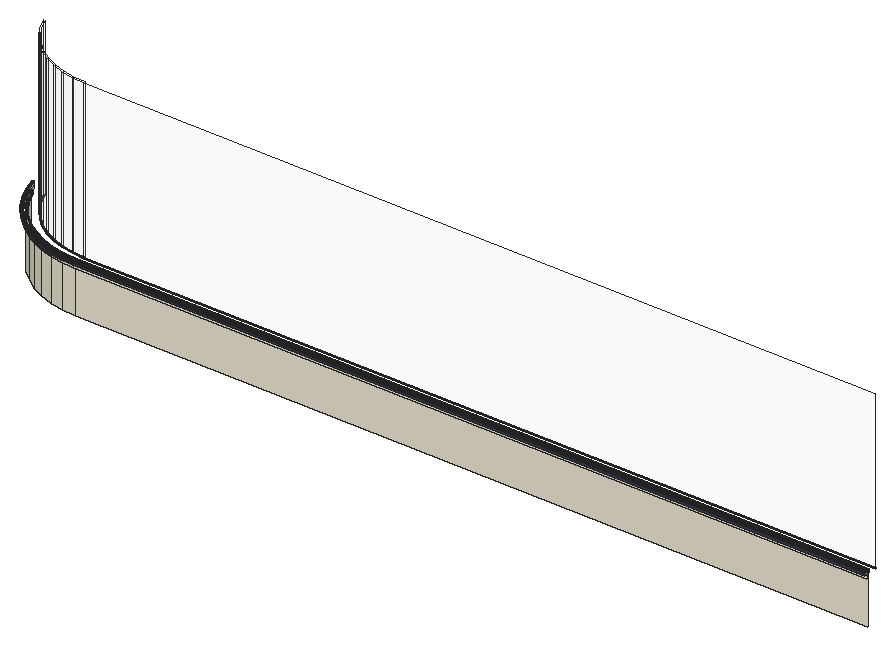
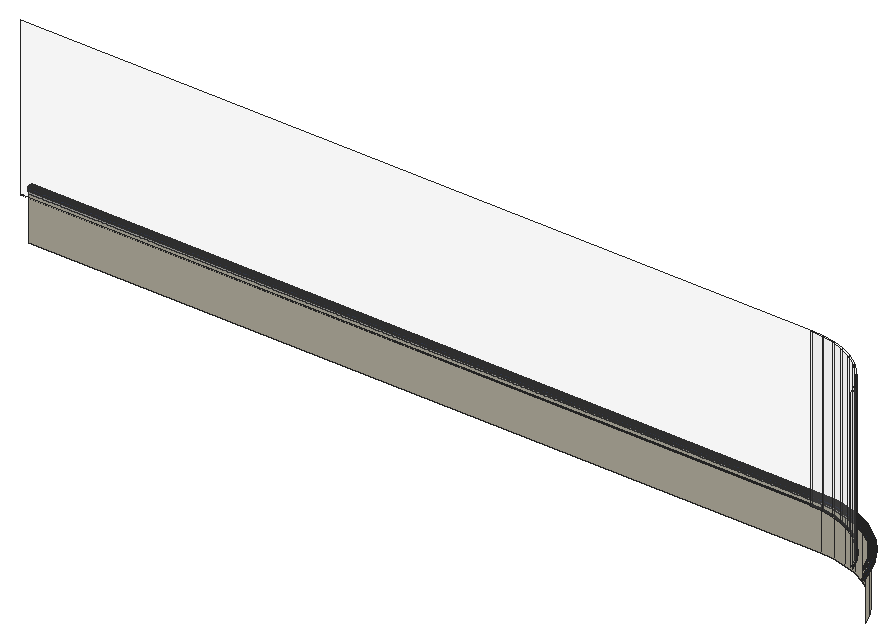
# SketchUp Ruby script. Lengths in inches.
U = 1.inch
M = Sketchup.active_model
def pt(a) = Geom::Point3d.new(a.map { |v| v * U })
def face(e, loops, mat)
  f = e.add_face(loops[0].map { |a| pt(a) })
  loops[1..].each { |l| e.add_face(l.map { |a| pt(a) }).erase! }
  f.material = f.back_material = mat if mat
  f
end
# faces: each face lists its corners as indices into pts; further lists are holes
def faces(e, pts, list, mat = nil) = list.each { |f| face(e, (f[0].is_a?(Array) ? f : [f]).map { |l| l.map { |i| pts[i] } }, mat) }
# xy, xz, yz: faces in a plane at the given z, y or x. An outline is a flat list of corners, or four numbers for a rectangle; further outlines are holes
def ring(l) = l.size == 4 ? [[l[0], l[1]], [l[2], l[1]], [l[2], l[3]], [l[0], l[3]]] : l.each_slice(2).to_a
def flat(e, list, mat, &to3) = list.each { |f| face(e, (f[0].is_a?(Array) ? f : [f]).map { |l| ring(l).map { |u, v| to3.(u, v) } }, mat) }
def xy(e, z, list, mat = nil) = flat(e, list, mat) { |x, y| [x, y, z] }
def xz(e, y, list, mat = nil) = flat(e, list, mat) { |x, z| [x, y, z] }
def yz(e, x, list, mat = nil) = flat(e, list, mat) { |y, z| [x, y, z] }
def lines(e, pts, list) = list.each { |a, b| e.add_line(pt(pts[a]), pt(pts[b])) }
# prism: a flat outline (further loops are holes) pulled along v
def prism(e, loops, v, mat = nil)
  f = face(e, loops, mat); d = Geom::Vector3d.new(v.map { |x| x * U })
  f.pushpull(f.normal.samedirection?(d) ? d.length : -d.length)
end
def box(e, o, s, mat = nil) = prism(e, [[o, [o[0] + s[0], o[1], o[2]], [o[0] + s[0], o[1] + s[1], o[2]], [o[0], o[1] + s[1], o[2]]]], [0, 0, s[2]], mat)
def at(x, y, z, deg = 0) = Geom::Transformation.translation(pt([x, y, z])) * Geom::Transformation.rotation(ORIGIN, Z_AXIS, deg.degrees)
def axes(o, x, y, z) = Geom::Transformation.new([*x, 0, *y, 0, *z, 0, *pt(o).to_a, 1])
def part(name) = M.definitions.add(name)
# library, detail: a bought-in or finely detailed component or shape, given as its bounding box
def library(name, o, s) = part(name).tap { |d| box(d.entities, o, s) }
def detail(e, o, s) = box(e.add_group.entities, o, s)
def put(e, d, t, mat = nil) = e.add_instance(d, t).tap { |i| i.material = mat if mat }
def group(e, t, mat = nil) = e.add_group.tap { |g| g.transformation = t; g.material = mat if mat }.entities
root = M.entities
M.materials.add("0360 AP 9644 Monsoon Midnight-N").color = [56, 67, 95]
M.materials.add("0905 AP 7844 MILD YELLOW").color = [242, 237, 215]
M.materials.add("Glass Clear 001").color = [246, 246, 246]
M.materials["Glass Clear 001"].alpha = 0.1
xz(root,29.01,[[57,132.5625,238.5625,132.625],[57,132.625,238.5625,132.8125]],"0360 AP 9644 Monsoon Midnight-N")
xz(root,29.09,[[57,132.5625,238.5625,132.625]])
xz(root,29.09,[[57,132,238.5625,132.5625],[57,132.625,238.5625,132.8125]],"0360 AP 9644 Monsoon Midnight-N")
xz(root,29.45,[[57,132,238.5625,132.625]])
xz(root,29.45,[[57,132.625,238.5625,132.8125]],"0360 AP 9644 Monsoon Midnight-N")
xz(root,29.45,[[57,131.3125,238.5625,132]],"0905 AP 7844 MILD YELLOW")
xz(root,29.53,[[57,132.625,238.5625,132.8125]],"0360 AP 9644 Monsoon Midnight-N")
xz(root,29.9375,[[57,131.3125,238.5625,132.625]])
xz(root,29.9375,[[57,132.625,238.5625,132.8125]],"0360 AP 9644 Monsoon Midnight-N")
xz(root,29.9375,[[57,121.25,238.5625,131.3125]],"0905 AP 7844 MILD YELLOW")
xz(root,30.29,[[57,132,238.5625,132.1875],[57,132.1875,238.5625,132.625],[57,132.625,238.5625,132.8125]],"0360 AP 9644 Monsoon Midnight-N")
xz(root,32.3125,[[57,132,238.5625,132.1875]],"0360 AP 9644 Monsoon Midnight-N")
xz(root,32.3125,[[57,132.1875,238.5625,168]],"Glass Clear 001")
p = [[57,29.9375,121.25],[57,29.9375,131.3125],[53.87,30.14,131.3125],[53.87,30.14,121.25],[50.79,30.76,131.3125],[50.79,30.76,121.25],
  [47.82,31.76,131.3125],[47.82,31.76,121.25],[45,33.15,131.3125],[45,33.15,121.25],[42.39,34.9,131.3125],[42.39,34.9,121.25],
  [40.03,36.97,131.3125],[40.03,36.97,121.25],[37.96,39.33,131.3125],[37.96,39.33,121.25],[36.22,41.9375,131.3125],[36.22,41.9375,121.25],
  [34.83,44.75,131.3125],[34.83,44.75,121.25],[57,29.45,132],[53.8,29.65,132],[53.8,29.65,131.3125],[57,29.45,131.3125],
  [50.66,30.28,132],[50.66,30.28,131.3125],[57,29.9375,132.625],[53.87,30.14,132.625],[50.79,30.76,132.625],[47.63,31.31,132],
  [47.63,31.31,131.3125],[47.82,31.76,132.625],[44.75,32.73,132],[44.75,32.73,131.3125],[45,33.15,132.625],[42.09,34.51,132],
  [42.09,34.51,131.3125],[42.39,34.9,132.625],[39.68,36.62,132],[39.68,36.62,131.3125],[40.03,36.97,132.625],[37.57,39.03,132],
  [37.57,39.03,131.3125],[37.96,39.33,132.625],[35.79,41.69,132],[35.79,41.69,131.3125],[36.22,41.9375,132.625],[34.37,44.56,132],
  [34.37,44.56,131.3125],[34.83,44.75,132.625],[33.34,47.6,132],[33.34,47.6,131.3125],[53.76,29.31,132],[57,29.09,132],
  [57,29.09,132.5625],[53.76,29.31,132.5625],[50.57,29.9375,132],[50.57,29.9375,132.5625],[53.8,29.65,132.625],[57,29.45,132.625],
  [50.66,30.28,132.625],[47.49,30.98,132],[47.49,30.98,132.5625],[47.63,31.31,132.625],[57,30.29,132],[53.91,30.49,132],
  [53.91,30.49,132.1875],[57,30.29,132.1875],[50.88,31.1,132],[50.88,31.1,132.1875],[44.58,32.42,132],[44.58,32.42,132.5625],
  [47.95,32.09,132],[47.95,32.09,132.1875],[44.75,32.73,132.625],[45.18,33.46,132],[45.18,33.46,132.1875],[54.18,32.5,132],
  [57,32.3125,132],[57,32.3125,132.1875],[54.18,32.5,132.1875],[41.875,34.23,132],[41.875,34.23,132.5625],[51.4,33.05,132],
  [51.4,33.05,132.1875],[42.09,34.51,132.625],[57,32.69,132],[54.23,32.87,132],[54.23,32.87,168],[57,32.69,168],
  [51.5,33.41,132],[51.5,33.41,168],[48.72,33.96,132],[48.72,33.96,132.1875],[48.87,34.31,132],[48.87,34.31,168],
  [42.6,35.18,132],[42.6,35.18,132.1875],[46.1875,35.21,132],[46.1875,35.21,132.1875],[39.43,36.37,132],[39.43,36.37,132.5625],
  [46.375,35.54,132],[46.375,35.54,168],[39.68,36.62,132.625],[40.28,37.22,132],[40.28,37.22,132.1875],[43.84,36.78,132],
  [43.84,36.78,132.1875],[44.07,37.08,132],[44.07,37.08,168],[37.29,38.8125,132],[37.29,38.8125,132.5625],[37.57,39.03,132.625],
  [41.71,38.65,132],[41.71,38.65,132.1875],[41.98,38.91,132],[41.98,38.91,168],[38.24,39.54,132],[38.24,39.54,132.1875],
  [39.84,40.77,132],[39.84,40.77,132.1875],[35.48,41.51,132],[35.48,41.51,132.5625],[40.14,41,132],[40.14,41,168],
  [35.79,41.69,132.625],[36.52,42.11,132],[36.52,42.11,132.1875],[38.27,43.125,132],[38.27,43.125,132.1875],[38.6,43.3125,132],
  [38.6,43.3125,168],[34.05,44.43,132],[34.05,44.43,132.5625],[34.37,44.56,132.625],[35.15,44.89,132],[35.15,44.89,132.1875],
  [37.02,45.66,132],[37.02,45.66,132.1875],[37.37,45.81,132],[37.37,45.81,168],[33,47.51,132],[33,47.51,132.5625],
  [33.34,47.6,132.625],[57,30.29,132.625],[53.91,30.49,132.625],[50.88,31.1,132.625],[47.95,32.09,132.625],[45.18,33.46,132.625],
  [54.18,32.5,168],[57,32.3125,168],[51.4,33.05,168],[48.72,33.96,168],[42.6,35.18,132.625],[46.1875,35.21,168],
  [40.28,37.22,132.625],[43.84,36.78,168],[41.71,38.65,168],[38.24,39.54,132.625],[39.84,40.77,168],[36.52,42.11,132.625],
  [38.27,43.125,168],[35.15,44.89,132.625],[37.02,45.66,168],[53.75,29.23,132.5625],[57,29.01,132.5625],[57,29.01,132.625],
  [53.75,29.23,132.625],[57,29.01,132.8125],[53.75,29.23,132.8125],[53.76,29.31,132.625],[57,29.09,132.625],[53.76,29.31,132.8125],
  [57,29.09,132.8125],[50.55,29.86,132.5625],[50.55,29.86,132.625],[50.55,29.86,132.8125],[50.57,29.9375,132.625],[50.57,29.9375,132.8125],
  [53.8,29.65,132.8125],[57,29.45,132.8125],[57,29.53,132.625],[53.8125,29.73,132.625],[53.8125,29.73,132.8125],[57,29.53,132.8125],
  [50.66,30.28,132.8125],[50.68,30.36,132.625],[50.68,30.36,132.8125],[47.46,30.91,132.5625],[47.46,30.91,132.625],[47.46,30.91,132.8125],
  [47.49,30.98,132.625],[47.49,30.98,132.8125],[53.87,30.14,132.8125],[57,29.9375,132.8125],[50.79,30.76,132.8125],[47.63,31.31,132.8125],
  [53.91,30.49,132.8125],[57,30.29,132.8125],[47.66,31.38,132.625],[47.66,31.38,132.8125],[50.88,31.1,132.8125],[47.82,31.76,132.8125],
  [44.54,32.35,132.5625],[44.54,32.35,132.625],[44.54,32.35,132.8125],[44.58,32.42,132.625],[44.58,32.42,132.8125],[47.95,32.09,132.8125],
  [44.75,32.73,132.8125],[44.79,32.8,132.625],[44.79,32.8,132.8125],[45,33.15,132.8125],[45.18,33.46,132.8125],[41.83,34.16,132.5625],
  [41.83,34.16,132.625],[41.83,34.16,132.8125],[41.875,34.23,132.625],[41.875,34.23,132.8125],[42.09,34.51,132.8125],[42.14,34.57,132.625],
  [42.14,34.57,132.8125],[42.39,34.9,132.8125],[42.6,35.18,132.8125],[39.375,36.3125,132.5625],[39.375,36.3125,132.625],[39.375,36.3125,132.8125],
  [39.43,36.37,132.625],[39.43,36.37,132.8125],[39.68,36.62,132.8125],[39.74,36.68,132.625],[39.74,36.68,132.8125],[40.03,36.97,132.8125],
  [40.28,37.22,132.8125],[37.23,38.76,132.5625],[37.23,38.76,132.625],[37.23,38.76,132.8125],[37.29,38.8125,132.625],[37.29,38.8125,132.8125],
  [37.57,39.03,132.8125],[37.63,39.08,132.625],[37.63,39.08,132.8125],[37.96,39.33,132.8125],[38.24,39.54,132.8125],[35.41,41.47,132.5625],
  [35.41,41.47,132.625],[35.41,41.47,132.8125],[35.48,41.51,132.625],[35.48,41.51,132.8125],[35.79,41.69,132.8125],[35.86,41.73,132.625],
  [35.86,41.73,132.8125],[36.22,41.9375,132.8125],[36.52,42.11,132.8125],[33.97,44.4,132.5625],[33.97,44.4,132.625],[33.97,44.4,132.8125],
  [34.05,44.43,132.625],[34.05,44.43,132.8125],[34.37,44.56,132.8125],[34.45,44.6,132.625],[34.45,44.6,132.8125],[34.83,44.75,132.8125],
  [35.15,44.89,132.8125],[32.92,47.49,132.5625],[32.92,47.49,132.625],[32.92,47.49,132.8125],[33,47.51,132.625],[33,47.51,132.8125],
  [33.34,47.6,132.8125]]
faces(root,p,[[0,1,2,3],[3,2,4,5],[5,4,6,7],[7,6,8,9],[9,8,10,11],[11,10,12,13],[13,12,14,15],[15,14,16,17],
  [17,16,18,19],[20,21,22,23],[21,24,25,22],[24,29,30,25],[29,32,33,30],[32,35,36,33],[35,38,39,36],[38,41,42,39],
  [41,44,45,42],[44,47,48,45],[47,50,51,48]],"0905 AP 7844 MILD YELLOW")
faces(root,p,[[1,26,27,2],[2,27,28,4],[4,28,31,6],[6,31,34,8],[8,34,37,10],[10,37,40,12],[12,40,43,14],[14,43,46,16],
  [16,46,49,18],[20,21,58,59],[21,24,60,58],[24,29,63,60],[29,32,74,63],[32,35,85,74],[35,38,104,85],[38,41,113,104],
  [41,44,126,113],[44,47,135,126],[47,50,144,135],[54,55,171,172],[55,57,178,171],[57,62,192,178],[62,71,207,192],[71,82,218,207],
  [82,101,228,218],[101,112,238,228],[112,123,248,238],[123,134,258,248],[134,143,268,258]])
faces(root,p,[[52,53,54,55],[56,52,55,57],[61,56,57,62],[64,65,66,67],[65,68,69,66],[70,61,62,71],[68,72,73,69],[72,75,76,73],
  [77,78,79,80],[81,70,71,82],[83,77,80,84],[92,83,84,93],[75,96,97,76],[98,92,93,99],[100,81,82,101],[96,105,106,97],
  [107,98,99,108],[111,100,101,112],[114,107,108,115],[105,118,119,106],[120,114,115,121],[122,111,112,123],[118,127,128,119],[129,120,121,130],
  [133,122,123,134],[127,136,137,128],[138,129,130,139],[142,133,134,143],[145,67,66,146],[146,66,69,147],[147,69,73,148],[148,73,76,149],
  [149,76,97,154],[154,97,106,156],[156,106,119,159],[159,119,128,161],[161,128,137,163],[165,166,167,168],[168,167,169,170],[172,171,173,174],
  [175,165,168,176],[176,168,170,177],[171,178,179,173],[59,58,180,181],[182,183,184,185],[58,60,186,180],[183,187,188,184],[189,175,176,190],
  [190,176,177,191],[178,192,193,179],[26,27,194,195],[27,28,196,194],[60,63,197,186],[145,146,198,199],[187,200,201,188],[146,147,202,198],
  [28,31,203,196],[204,189,190,205],[205,190,191,206],[192,207,208,193],[147,148,209,202],[63,74,210,197],[200,211,212,201],[31,34,213,203],
  [148,149,214,209],[215,204,205,216],[216,205,206,217],[207,218,219,208],[74,85,220,210],[211,221,222,212],[34,37,223,213],[149,154,224,214],
  [225,215,216,226],[226,216,217,227],[218,228,229,219],[85,104,230,220],[221,231,232,222],[37,40,233,223],[154,156,234,224],[235,225,226,236],
  [236,226,227,237],[228,238,239,229],[104,113,240,230],[231,241,242,232],[40,43,243,233],[156,159,244,234],[245,235,236,246],[246,236,237,247],
  [238,248,249,239],[113,126,250,240],[241,251,252,242],[43,46,253,243],[159,161,254,244],[255,245,246,256],[256,246,247,257],[248,258,259,249],
  [126,135,260,250],[251,261,262,252],[46,49,263,253],[161,163,264,254],[265,255,256,266],[266,256,257,267],[258,268,269,259],[135,144,270,260]],"0360 AP 9644 Monsoon Midnight-N")
faces(root,p,[[86,87,88,89],[87,90,91,88],[90,94,95,91],[94,102,103,95],[102,109,110,103],[109,116,117,110],[116,124,125,117],[124,131,132,125],
  [131,140,141,132],[150,80,79,151],[152,84,80,150],[153,93,84,152],[155,99,93,153],[157,108,99,155],[158,115,108,157],[160,121,115,158],
  [162,130,121,160],[164,139,130,162]],"Glass Clear 001")
